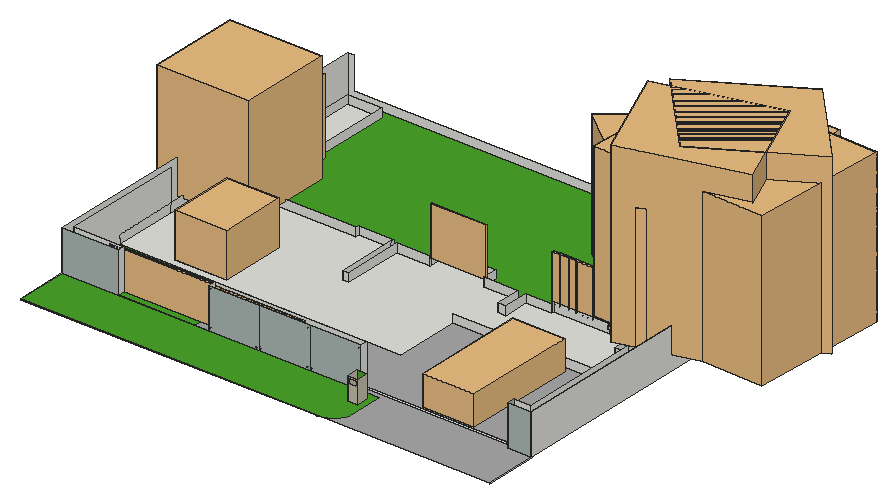
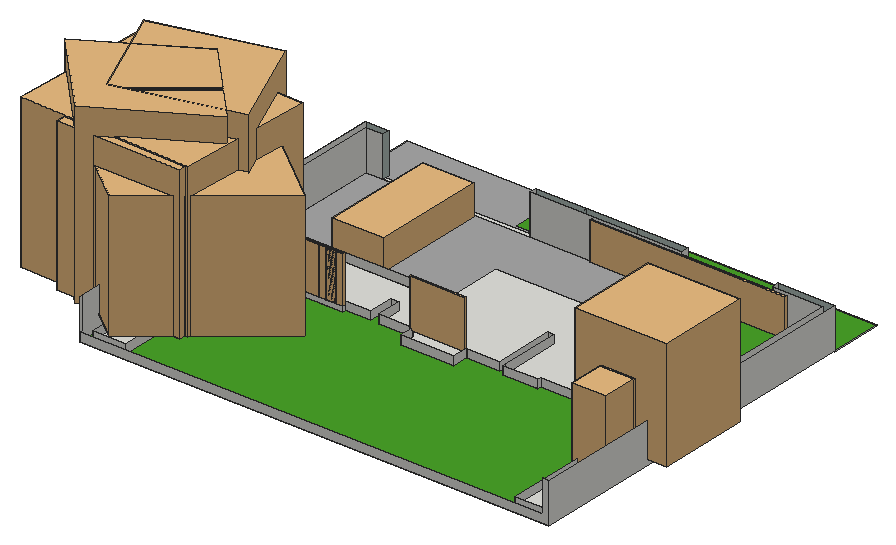
# SketchUp Ruby script. Lengths in inches.
U = 1.inch
M = Sketchup.active_model
def pt(a) = Geom::Point3d.new(a.map { |v| v * U })
def face(e, loops, mat)
  f = e.add_face(loops[0].map { |a| pt(a) })
  loops[1..].each { |l| e.add_face(l.map { |a| pt(a) }).erase! }
  f.material = f.back_material = mat if mat
  f
end
# faces: each face lists its corners as indices into pts; further lists are holes
def faces(e, pts, list, mat = nil) = list.each { |f| face(e, (f[0].is_a?(Array) ? f : [f]).map { |l| l.map { |i| pts[i] } }, mat) }
# xy, xz, yz: faces in a plane at the given z, y or x. An outline is a flat list of corners, or four numbers for a rectangle; further outlines are holes
def ring(l) = l.size == 4 ? [[l[0], l[1]], [l[2], l[1]], [l[2], l[3]], [l[0], l[3]]] : l.each_slice(2).to_a
def flat(e, list, mat, &to3) = list.each { |f| face(e, (f[0].is_a?(Array) ? f : [f]).map { |l| ring(l).map { |u, v| to3.(u, v) } }, mat) }
def xy(e, z, list, mat = nil) = flat(e, list, mat) { |x, y| [x, y, z] }
def xz(e, y, list, mat = nil) = flat(e, list, mat) { |x, z| [x, y, z] }
def yz(e, x, list, mat = nil) = flat(e, list, mat) { |y, z| [x, y, z] }
def lines(e, pts, list) = list.each { |a, b| e.add_line(pt(pts[a]), pt(pts[b])) }
# prism: a flat outline (further loops are holes) pulled along v
def prism(e, loops, v, mat = nil)
  f = face(e, loops, mat); d = Geom::Vector3d.new(v.map { |x| x * U })
  f.pushpull(f.normal.samedirection?(d) ? d.length : -d.length)
end
def box(e, o, s, mat = nil) = prism(e, [[o, [o[0] + s[0], o[1], o[2]], [o[0] + s[0], o[1] + s[1], o[2]], [o[0], o[1] + s[1], o[2]]]], [0, 0, s[2]], mat)
def at(x, y, z, deg = 0) = Geom::Transformation.translation(pt([x, y, z])) * Geom::Transformation.rotation(ORIGIN, Z_AXIS, deg.degrees)
def axes(o, x, y, z) = Geom::Transformation.new([*x, 0, *y, 0, *z, 0, *pt(o).to_a, 1])
def part(name) = M.definitions.add(name)
# library, detail: a bought-in or finely detailed component or shape, given as its bounding box
def library(name, o, s) = part(name).tap { |d| box(d.entities, o, s) }
def detail(e, o, s) = box(e.add_group.entities, o, s)
def put(e, d, t, mat = nil) = e.add_instance(d, t).tap { |i| i.material = mat if mat }
def group(e, t, mat = nil) = e.add_group.tap { |g| g.transformation = t; g.material = mat if mat }.entities
root = M.entities
M.materials.add("Material~3").color = [123, 113, 102]
M.materials.add("[0116_Lavender]").color = [73, 163, 41]
M.materials.add("[0132_LightGray]").color = [169, 169, 169]
M.materials.add("[Slate]").color = [172, 186, 182]
M.materials.add("[Tile Canvas]").color = [199, 192, 173]
M.materials.add("[Tile Grey]").color = [168, 168, 168]
c1 = library("Floor plant",[-5.56,-16.3125,0.81],[76.88,76.71,92.33])
c2 = library("Potted broadleaf plant",[-29.7,0,-10.87],[31.67,38.52,72.45])
c3 = library("Sem+nome (1)",[20.77,3.52,-2.22],[96.42,122.82,82.56])
c4 = library("Sliding Gate",[0,0,0],[194.88,4.13,70.58])
c5 = library("3 door",[0,0,0],[74.8,3.9375,43.31])
c6 = library("3DGeom~4_Defintion",[362.52,-15.59,12.6],[288.85,70.11,1000])
c7 = library("BMW 8 Series M850i 2019",[-14.25,0.77,-0.16],[87.38,190.63,50.87])
c8 = library("Group\#65",[-33.32,-34.9375,32.67],[162.87,159.66,128.34])
c9 = library("Group\#81",[-10.45,-6.67,0],[121.7,116.61,164.95])
c10 = library("Group\#82",[-10.45,-6.67,0],[121.7,116.61,164.95])
c11 = library("Group\#69",[-10.45,-6.67,0],[121.7,116.61,164.95])
c12 = library("Group\#83",[-33.32,-34.9375,32.67],[162.87,159.66,128.34])
c13 = library("Group\#64",[-33.32,-34.9375,81.35],[162.87,159.66,79.66])
c14 = library("Group\#80",[-33.32,-34.9375,77.91],[162.87,159.66,83.1])
c15 = part("Palem Elek")
put(c15.entities,c8,axes([92.2,20.3,-29.73],[0.70711,0.70711,0],[-0.70711,0.70711,0],[0,0,0.91208]))
put(c15.entities,c9,axes([60.27,20.78,0],[1,0,0],[0,1,0],[0,0,0.85762]))
put(c15.entities,c10,at(25.45,60.83,0,-53.5))
put(c15.entities,c11,at(84.4375,135.48,0,-161.4))
put(c15.entities,c12,axes([38.54,105.7,-36.19],[-0.04013,-0.99919,0],[0.99919,-0.04013,0],[0,0,1.11001]))
put(c15.entities,c13,axes([57.15,96.51,-54.45],[-0.02003,-0.49872,0.02965],[0.4996,-0.02007,0],[0.00123,0.03065,0.51628]))
put(c15.entities,c14,axes([74.94,50.39,-54.06],[0.40095,0.29715,0.03075],[-0.29654,0.38966,0.10114],[0.04012,-0.11026,0.54246]))
c16 = part("palem elek\#1")
put(c16.entities,c15,at(-81.14,-74.56,-0.83))
c17 = part("Coqueiro")
put(c17.entities,c16,axes([83.17,89.39,9.5625],[0,1.1016,0],[-1.377,0,0],[0,0,1.39284]))
xy(root,-10.51,[[2596.56,498.28,2873.37,505.1],[[2048.43,611.53,2048.43,1146.63,2112.0625,1146.63,2112.0625,732.28,2123,732.28,2123,845.35,2305.05,845.35,2305.05,851.0625,2370.42,851.0625,2370.42,732.28,2381.36,732.28,2381.36,845.35,2444.05,845.35,2444.05,874.25,2544.33,874.25,2544.33,845.35,2608.61,845.35,2608.61,798.41,2623.94,798.41,2623.94,845.35,2671.4,845.35,2671.4,851.0625,2840.8125,851.0625,2840.8125,1146.63,2904.07,1146.63,2904.07,732.28,2576.35,732.28,2576.35,611.53],[2825.48,801.78,2840.8125,845.35]]])
xy(root,-10.51,[[[2036.8125,393.78,2607.06,393.78,2610.09,394.71,2613.02,395.9,2615.84,397.35,2618.51,399.04,2621.03,400.97,2623.36,403.1,2625.5,405.44,2627.42,407.96,2629.11,410.63,2630.5625,413.45,2631.76,416.38,2632.68,419.41,2632.68,491.47,2596.56,491.47,2596.56,505.1,2311.71,505.1,2311.71,491.47,2142.71,491.47,2142.71,505.1,2048.43,505.1,2048.43,1146.63,2112.0625,1146.63,2112.0625,732.28,2123,732.28,2123,845.35,2305.05,845.35,2305.05,851.0625,2370.42,851.0625,2370.42,732.28,2381.36,732.28,2381.36,845.35,2444.05,845.35,2444.05,874.25,2544.33,874.25,2544.33,845.35,2608.61,845.35,2608.61,798.41,2623.94,798.41,2623.94,845.35,2671.4,845.35,2671.4,851.0625,2840.8125,851.0625,2840.8125,1146.63,2904.07,1146.63,2904.07,505.1,2873.37,505.1,2873.37,491.47,2916.0625,491.47,2916.0625,1160.85,2036.8125,1160.85],[2602.58,453.42,2621.02,475.99]],[2142.71,491.47,2286.14,491.47,2291.35,611.53,2048.43,611.53,2048.43,505.1,2142.71,505.1]],"[0116_Lavender]")
xy(root,-10.51,[[2607.06,393.78,2916.0625,393.78,2916.0625,491.47,2873.37,491.47,2873.37,498.28,2596.56,498.28,2596.56,491.47,2632.68,491.47,2632.68,419.41,2631.76,416.38,2630.5625,413.45,2629.11,410.63,2627.42,407.96,2625.5,405.44,2623.36,403.1,2621.03,400.97,2618.51,399.04,2615.84,397.35,2613.02,395.9,2610.09,394.71],[2286.14,491.47,2311.71,491.47,2311.71,505.1,2904.07,505.1,2904.07,732.28,2576.35,732.28,2576.35,611.53,2291.35,611.53]],"[Tile Grey]")
xz(root,393.78,[[2036.8125,-12.6875,2311.71,-12.6875,2596.56,-10.51,2036.8125,-10.51]])
xz(root,453.42,[[[2602.58,-10.51,2621.02,32.74],[2604.93,19.53,2619.05,29.34]]],"[Tile Canvas]")
xz(root,475.99,[[2602.58,-10.51,2621.02,32.74]],"[0116_Lavender]")
xz(root,491.47,[[2142.71,-12.6875,2311.71,-10.51]])
xz(root,491.47,[[2402.92,-7.89,2403.41,-7.82,2403.86,-7.63,2404.25,-7.34,2404.55,-6.95,2404.73,-6.5,2404.8,-6.01,2404.73,-5.52,2404.55,-5.07,2404.25,-4.68,2403.86,-4.39,2403.41,-4.2,2402.92,-4.14,2402.4375,-4.2,2401.99,-4.39,2401.6,-4.68,2401.3,-5.07,2401.11,-5.52,2401.05,-6.01,2401.11,-6.5,2401.3,-6.95,2401.6,-7.34,2401.99,-7.63,2402.4375,-7.82],[2497.875,-7.89,2498.36,-7.82,2498.8125,-7.63,2499.2,-7.34,2499.5,-6.95,2499.69,-6.5,2499.75,-6.01,2499.69,-5.52,2499.5,-5.07,2499.2,-4.68,2498.8125,-4.39,2498.36,-4.2,2497.875,-4.14,2497.39,-4.2,2496.9375,-4.39,2496.55,-4.68,2496.25,-5.07,2496.0625,-5.52,2496,-6.01,2496.0625,-6.5,2496.25,-6.95,2496.55,-7.34,2496.9375,-7.63,2497.39,-7.82],[2592.82,-7.89,2593.31,-7.82,2593.76,-7.63,2594.15,-7.34,2594.45,-6.95,2594.64,-6.5,2594.7,-6.01,2594.64,-5.52,2594.45,-5.07,2594.15,-4.68,2593.76,-4.39,2593.31,-4.2,2592.82,-4.14,2592.34,-4.2,2591.89,-4.39,2591.5,-4.68,2591.2,-5.07,2591.01,-5.52,2590.95,-6.01,2591.01,-6.5,2591.2,-6.95,2591.5,-7.34,2591.89,-7.63,2592.34,-7.82],[2315.19,-6.41,2315.68,-6.4,2316.15,-6.26,2316.57,-6.01,2316.9,-5.66,2317.14,-5.23,2317.25,-4.75,2317.24,-4.26,2317.1,-3.79,2316.85,-3.375,2316.49,-3.04,2316.07,-2.8,2315.59,-2.6875,2315.1,-2.7,2314.63,-2.84,2314.21,-3.09,2313.875,-3.45,2313.64,-3.875,2313.53,-4.35,2313.54,-4.84,2313.68,-5.31,2313.93,-5.73,2314.28,-6.07,2314.71,-6.3],[2410.14,-6.41,2410.63,-6.4,2411.1,-6.26,2411.52,-6.01,2411.86,-5.66,2412.09,-5.23,2412.2,-4.75,2412.19,-4.26,2412.05,-3.79,2411.8,-3.375,2411.45,-3.04,2411.02,-2.8,2410.54,-2.6875,2410.05,-2.7,2409.58,-2.84,2409.16,-3.09,2408.83,-3.45,2408.59,-3.875,2408.48,-4.35,2408.49,-4.84,2408.625,-5.31,2408.88,-5.73,2409.24,-6.07,2409.67,-6.3],
  [2505.09,-6.41,2505.58,-6.4,2506.05,-6.26,2506.47,-6.01,2506.81,-5.66,2507.04,-5.23,2507.16,-4.75,2507.14,-4.26,2507.01,-3.79,2506.75,-3.375,2506.4,-3.04,2505.97,-2.8,2505.49,-2.6875,2505,-2.7,2504.53,-2.84,2504.11,-3.09,2503.78,-3.45,2503.54,-3.875,2503.43,-4.35,2503.4375,-4.84,2503.58,-5.31,2503.83,-5.73,2504.1875,-6.07,2504.62,-6.3]],"[0132_LightGray]")
xz(root,491.47,[[2036.8125,-12.6875,2142.71,65.1875],[[2311.71,-12.6875,2596.56,-10.51,2596.56,65.1875,2311.71,65.1875],[2402.92,-7.89,2402.4375,-7.82,2401.99,-7.63,2401.6,-7.34,2401.3,-6.95,2401.11,-6.5,2401.05,-6.01,2401.11,-5.52,2401.3,-5.07,2401.6,-4.68,2401.99,-4.39,2402.4375,-4.2,2402.92,-4.14,2403.41,-4.2,2403.86,-4.39,2404.25,-4.68,2404.55,-5.07,2404.73,-5.52,2404.8,-6.01,2404.73,-6.5,2404.55,-6.95,2404.25,-7.34,2403.86,-7.63,2403.41,-7.82],[2497.875,-7.89,2497.39,-7.82,2496.9375,-7.63,2496.55,-7.34,2496.25,-6.95,2496.0625,-6.5,2496,-6.01,2496.0625,-5.52,2496.25,-5.07,2496.55,-4.68,2496.9375,-4.39,2497.39,-4.2,2497.875,-4.14,2498.36,-4.2,2498.8125,-4.39,2499.2,-4.68,2499.5,-5.07,2499.69,-5.52,2499.75,-6.01,2499.69,-6.5,2499.5,-6.95,2499.2,-7.34,2498.8125,-7.63,2498.36,-7.82],[2402.92,57.74,2402.4375,57.8,2401.99,57.99,2401.6,58.29,2401.3,58.68,2401.11,59.13,2401.05,59.61,2401.11,60.1,2401.3,60.55,2401.6,60.94,2401.99,61.24,2402.4375,61.43,2402.92,61.49,2403.41,61.43,2403.86,61.24,2404.25,60.94,2404.55,60.55,2404.73,60.1,2404.8,59.61,2404.73,59.13,2404.55,58.68,2404.25,58.29,2403.86,57.99,2403.41,57.8],[2497.875,57.74,2497.39,57.8,2496.9375,57.99,2496.55,58.29,2496.25,58.68,2496.0625,59.13,2496,59.61,2496.0625,60.1,2496.25,60.55,2496.55,60.94,2496.9375,61.24,2497.39,61.43,2497.875,61.49,2498.36,61.43,2498.8125,61.24,2499.2,60.94,2499.5,60.55,2499.69,60.1,2499.75,59.61,2499.69,59.13,2499.5,58.68,2499.2,58.29,2498.8125,57.99,2498.36,57.8],[2592.82,-7.89,2592.34,-7.82,2591.89,-7.63,2591.5,-7.34,2591.2,-6.95,2591.01,-6.5,2590.95,-6.01,2591.01,-5.52,2591.2,-5.07,2591.5,-4.68,2591.89,-4.39,2592.34,-4.2,2592.82,-4.14,2593.31,-4.2,2593.76,-4.39,2594.15,-4.68,2594.45,-5.07,2594.64,-5.52,2594.7,-6.01,2594.64,-6.5,2594.45,-6.95,2594.15,-7.34,2593.76,-7.63,2593.31,-7.82],[2592.82,57.74,2592.34,57.8,2591.89,57.99,2591.5,58.29,2591.2,58.68,2591.01,59.13,2590.95,59.61,2591.01,60.1,2591.2,60.55,2591.5,60.94,2591.89,61.24,2592.34,61.43,2592.82,61.49,2593.31,61.43,2593.76,61.24,2594.15,60.94,2594.45,60.55,2594.64,60.1,2594.7,59.61,2594.64,59.13,2594.45,58.68,2594.15,58.29,2593.76,57.99,2593.31,57.8],[2410.14,59.21,2409.67,59.33,2409.24,59.56,2408.88,59.9,2408.625,60.32,2408.49,60.78,2408.48,61.27,2408.59,61.75,2408.83,62.18,2409.16,62.53,2409.58,62.79,2410.05,62.93,2410.54,62.9375,2411.02,62.82,2411.45,62.59,2411.8,62.25,2412.05,61.83,2412.19,61.36,2412.2,60.875,2412.09,60.4,2411.86,59.97,2411.52,59.61,2411.1,59.36,2410.63,59.22],[2505.09,59.21,2504.62,59.33,2504.1875,59.56,2503.83,59.9,2503.58,60.32,2503.4375,60.78,2503.43,61.27,2503.54,61.75,2503.78,62.18,2504.11,62.53,2504.53,62.79,2505,62.93,2505.49,62.9375,2505.97,62.82,2506.4,62.59,2506.75,62.25,2507.01,61.83,2507.14,61.36,2507.16,60.875,2507.04,60.4,2506.81,59.97,2506.47,59.61,2506.05,59.36,2505.58,59.22],[2315.19,-6.41,2314.71,-6.3,2314.28,-6.07,2313.93,-5.73,2313.68,-5.31,2313.54,-4.84,2313.53,-4.35,2313.64,-3.875,2313.875,-3.45,2314.21,-3.09,2314.63,-2.84,2315.1,-2.7,2315.59,-2.6875,2316.07,-2.8,2316.49,-3.04,2316.85,-3.375,2317.1,-3.79,2317.24,-4.26,2317.25,-4.75,2317.14,-5.23,2316.9,-5.66,2316.57,-6.01,2316.15,-6.26,2315.68,-6.4],[2410.14,-6.41,2409.67,-6.3,2409.24,-6.07,2408.88,-5.73,2408.625,-5.31,2408.49,-4.84,2408.48,-4.35,2408.59,-3.875,2408.83,-3.45,2409.16,-3.09,2409.58,-2.84,2410.05,-2.7,2410.54,-2.6875,2411.02,-2.8,2411.45,-3.04,2411.8,-3.375,2412.05,-3.79,2412.19,-4.26,2412.2,-4.75,2412.09,-5.23,2411.86,-5.66,2411.52,-6.01,2411.1,-6.26,2410.63,-6.4],[2505.09,-6.41,2504.62,-6.3,2504.1875,-6.07,2503.83,-5.73,2503.58,-5.31,2503.4375,-4.84,2503.43,-4.35,2503.54,-3.875,2503.78,-3.45,2504.11,-3.09,2504.53,-2.84,2505,-2.7,2505.49,-2.6875,2505.97,-2.8,2506.4,-3.04,2506.75,-3.375,2507.01,-3.79,2507.14,-4.26,2507.16,-4.75,2507.04,-5.23,2506.81,-5.66,2506.47,-6.01,2506.05,-6.26,2505.58,-6.4],[2315.19,59.21,2314.71,59.33,2314.28,59.56,2313.93,59.9,2313.68,60.32,2313.54,60.78,2313.53,61.27,2313.64,61.75,2313.875,62.18,2314.21,62.53,2314.63,62.79,2315.1,62.93,2315.59,62.9375,2316.07,62.82,2316.49,62.59,2316.85,62.25,2317.1,61.83,2317.24,61.36,2317.25,60.875,2317.14,60.4,2316.9,59.97,2316.57,59.61,2316.15,59.36,2315.68,59.22]],[2873.37,-10.51,2916.0625,65.1875]],"[Slate]")
xz(root,505.1,[[2048.43,-10.51,2142.71,65.1875],[2311.71,-10.51,2596.56,65.1875],[2873.37,-10.51,2904.07,65.1875]])
xz(root,732.28,[[2112.0625,-10.51,2123,5.1875],[2370.42,-10.51,2381.36,5.1875],[2576.35,-10.51,2904.07,5.1875]])
xz(root,798.41,[[2608.61,-10.51,2623.94,5.1875]])
xz(root,801.78,[[2825.48,-10.51,2840.8125,5.1875]])
xz(root,845.35,[[2123,-10.51,2305.05,5.1875],[2381.36,-10.51,2444.05,5.1875],[2544.33,-10.51,2608.61,5.1875],[2623.94,-10.51,2671.4,5.1875],[2825.48,-10.51,2840.8125,5.1875],
  [2776.01,-0.125,2825.48,5.1875]])
xz(root,851.0625,[[2305.05,-10.51,2370.42,5.1875],[2671.4,-10.51,2776.01,5.1875],[2776.01,-10.51,2835.1,5.1875],[2835.1,-10.51,2840.8125,5.1875]])
xz(root,874.25,[[2444.05,-10.51,2544.33,5.1875]])
xz(root,1146.63,[[2048.43,-10.51,2112.0625,5.1875],[2840.8125,-10.51,2904.07,5.1875]])
xz(root,1160.85,[[2036.8125,-10.51,2036.8125,65.1875,2048.43,65.1875,2048.43,5.1875,2916.0625,5.1875,2916.0625,-10.51]])
yz(root,2036.8125,[[393.78,-12.6875,491.47,-10.51],[491.47,-10.51,1160.85,65.1875]])
yz(root,2048.43,[[505.1,-10.51,611.53,-10.51,611.53,5.1875,732.28,5.1875,732.28,65.1875,505.1,65.1875],[611.53,-10.51,732.28,5.1875],[732.28,-10.51,1146.63,5.1875]])
yz(root,2112.0625,[[732.28,-10.51,1146.63,5.1875]])
yz(root,2123,[[732.28,-10.51,845.35,5.1875]])
yz(root,2142.71,[[491.47,-10.51,505.1,65.1875]])
yz(root,2305.05,[[845.35,-10.51,851.0625,5.1875]])
yz(root,2311.71,[[491.47,-10.51,505.1,65.1875]])
yz(root,2370.42,[[732.28,-10.51,846.1,5.1875],[846.1,-10.51,851.0625,5.1875]])
yz(root,2381.36,[[732.28,-10.51,845.35,5.1875]])
yz(root,2444.05,[[845.35,-10.51,846.1,5.1875],[846.1,-10.51,874.25,5.1875]])
yz(root,2544.33,[[845.35,-10.51,846.1,5.1875],[846.1,-10.51,874.25,5.1875]])
yz(root,2596.56,[[491.47,-10.51,505.1,65.1875]])
yz(root,2602.58,[[453.42,-10.51,475.99,32.74]],"[Tile Canvas]")
yz(root,2608.61,[[798.41,-10.51,845.35,5.1875]])
yz(root,2621.02,[[453.42,-10.51,475.99,32.74]],"[Tile Canvas]")
yz(root,2623.94,[[798.41,-10.51,845.35,5.1875]])
yz(root,2671.4,[[845.35,-10.51,846.1,5.1875],[846.1,-10.51,851.0625,5.1875]])
yz(root,2776.01,[[845.35,-0.125,851.0625,5.1875]])
yz(root,2825.48,[[801.78,-10.51,845.35,5.1875]])
yz(root,2840.8125,[[801.78,-10.51,845.35,5.1875],[851.0625,-10.51,1146.63,5.1875]])
yz(root,2873.37,[[491.47,-10.51,505.1,65.1875]],"[Slate]")
yz(root,2904.07,[[505.1,-10.51,732.28,65.1875],[732.28,-10.51,1146.63,5.1875]])
yz(root,2916.0625,[[491.47,-10.51,1160.85,-10.51,1160.85,5.1875,1155.13,5.1875,1155.13,65.1875,491.47,65.1875]])
yz(root,2916.76,[[393.78,-12.6875,491.47,-10.51],[491.47,-10.51,1160.85,65.1875]])
p = [[2406.66,491.47,65.1875],[2406.66,491.47,-10.51],[2501.61,491.47,65.1875],[2501.61,491.47,-10.51]]
lines(root,p,[[0,1],[2,3]])
put(root,c1,axes([2011.23,797.14,-1],[2.24,0,0],[0,2.24,0],[0,0,2.24]))
put(root,c2,axes([2117.7,858.27,6.22],[2,0,0],[0,2,0],[0,0,2]))
put(root,c2,axes([2117.7,924.09,6.22],[2,0,0],[0,2,0],[0,0,2]))
put(root,c3,at(2128.83,611.53,-0.125))
put(root,c4,axes([2115.27,505.1,-10.51],[1.88,0,0],[0,1,0],[0,0,1]))
put(root,c5,axes([2444.05,846.14,1.53],[1.37387,0,0],[0,0.86071,0],[0,0,2.11056]))
put(root,c6,axes([2627.69,854.26,0.98],[0.11056,0,0],[0,-0.05859,0],[0,0,0.08734]),"Material~3")
put(root,c6,axes([2641.73,854.26,0.98],[0.11056,0,0],[0,-0.05859,0],[0,0,0.08734]),"Material~3")
put(root,c6,axes([2672.3125,854.26,0.98],[0.11056,0,0],[0,-0.05859,0],[0,0,0.08734]),"Material~3")
put(root,c7,axes([2780.05,720.81,-10.33],[-1.11,0,0],[0,-1.11,0],[0,0,1.11]))
put(root,c6,axes([2704,854.26,0.98],[0.11056,0,0],[0,-0.05859,0],[0,0,0.08734]),"Material~3")
put(root,c17,axes([2767.36,830.17,6.32],[1.44,0,0],[0,1.44,0],[0,0,1.44]))
